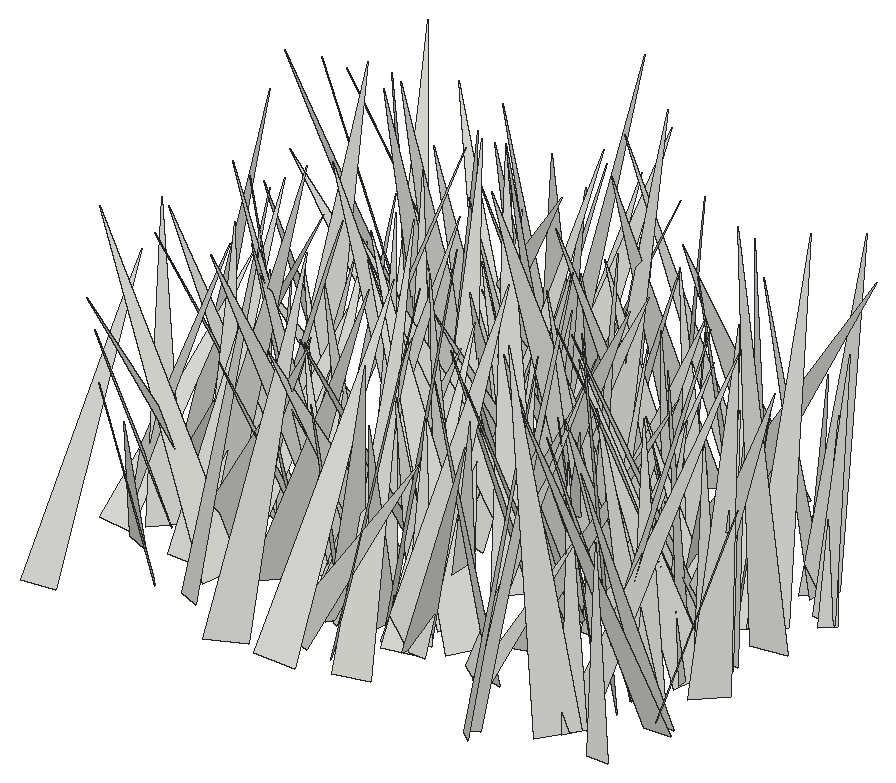
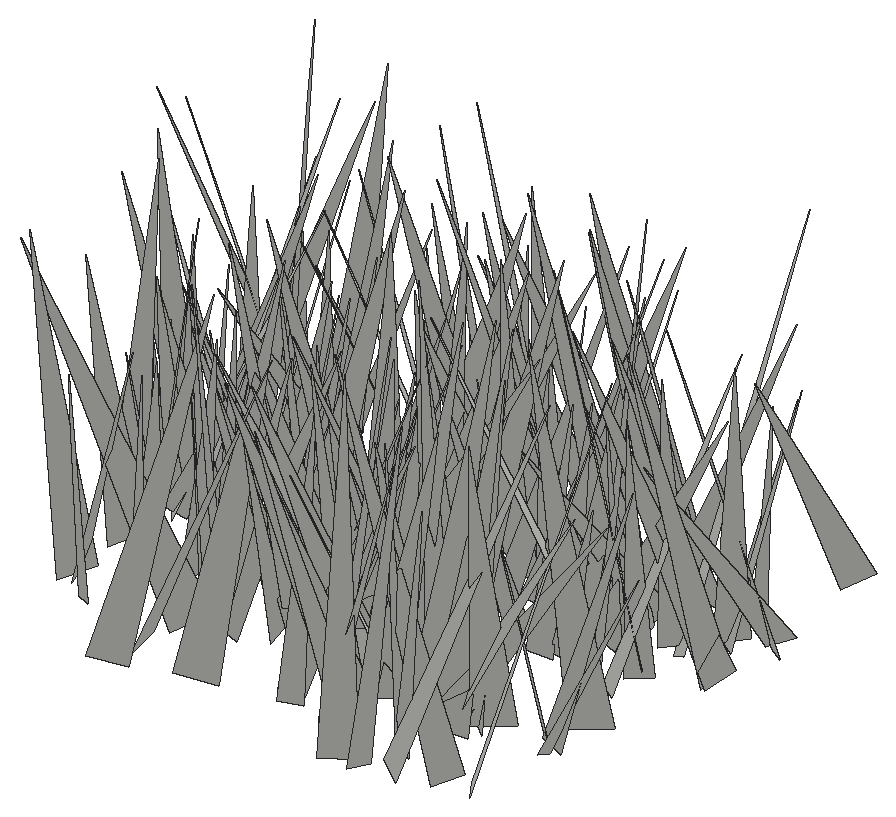
# SketchUp Ruby script. Lengths in inches.
U = 1.inch
M = Sketchup.active_model
def pt(a) = Geom::Point3d.new(a.map { |v| v * U })
def face(e, loops, mat)
  f = e.add_face(loops[0].map { |a| pt(a) })
  loops[1..].each { |l| e.add_face(l.map { |a| pt(a) }).erase! }
  f.material = f.back_material = mat if mat
  f
end
# faces: each face lists its corners as indices into pts; further lists are holes
def faces(e, pts, list, mat = nil) = list.each { |f| face(e, (f[0].is_a?(Array) ? f : [f]).map { |l| l.map { |i| pts[i] } }, mat) }
# xy, xz, yz: faces in a plane at the given z, y or x. An outline is a flat list of corners, or four numbers for a rectangle; further outlines are holes
def ring(l) = l.size == 4 ? [[l[0], l[1]], [l[2], l[1]], [l[2], l[3]], [l[0], l[3]]] : l.each_slice(2).to_a
def flat(e, list, mat, &to3) = list.each { |f| face(e, (f[0].is_a?(Array) ? f : [f]).map { |l| ring(l).map { |u, v| to3.(u, v) } }, mat) }
def xy(e, z, list, mat = nil) = flat(e, list, mat) { |x, y| [x, y, z] }
def xz(e, y, list, mat = nil) = flat(e, list, mat) { |x, z| [x, y, z] }
def yz(e, x, list, mat = nil) = flat(e, list, mat) { |y, z| [x, y, z] }
def lines(e, pts, list) = list.each { |a, b| e.add_line(pt(pts[a]), pt(pts[b])) }
# prism: a flat outline (further loops are holes) pulled along v
def prism(e, loops, v, mat = nil)
  f = face(e, loops, mat); d = Geom::Vector3d.new(v.map { |x| x * U })
  f.pushpull(f.normal.samedirection?(d) ? d.length : -d.length)
end
def box(e, o, s, mat = nil) = prism(e, [[o, [o[0] + s[0], o[1], o[2]], [o[0] + s[0], o[1] + s[1], o[2]], [o[0], o[1] + s[1], o[2]]]], [0, 0, s[2]], mat)
def at(x, y, z, deg = 0) = Geom::Transformation.translation(pt([x, y, z])) * Geom::Transformation.rotation(ORIGIN, Z_AXIS, deg.degrees)
def axes(o, x, y, z) = Geom::Transformation.new([*x, 0, *y, 0, *z, 0, *pt(o).to_a, 1])
def part(name) = M.definitions.add(name)
# library, detail: a bought-in or finely detailed component or shape, given as its bounding box
def library(name, o, s) = part(name).tap { |d| box(d.entities, o, s) }
def detail(e, o, s) = box(e.add_group.entities, o, s)
def put(e, d, t, mat = nil) = e.add_instance(d, t).tap { |i| i.material = mat if mat }
def group(e, t, mat = nil) = e.add_group.tap { |g| g.transformation = t; g.material = mat if mat }.entities
root = M.entities
c1 = part("fur_instance\#9")
p = [[0.8125,0,1.79],[0.67,-0.02,1.48],[0,-0.11,0],[0,0.11,0]]
faces(c1.entities,p,[[0,1,2,3]])
put(root,c1,axes([138.79,360.375,-27.1],[-2.84095,-2.72325,0.75235],[-2.80656,2.8428,-0.30791],[0.32453,0.74533,3.9233]))
put(root,c1,axes([145.17,360.07,-27.1],[2.54302,-4.52945,1.06711],[-4.23804,-1.75205,2.66287],[1.92189,2.12978,4.46004]))
put(root,c1,axes([158.66,360.0625,-27.1],[-0.06677,3.94377,1.582],[4.24655,0.00562,0.16522],[-0.15123,-1.5834,3.94087]))
put(root,c1,axes([143.4,358.59,-27.1],[5.43285,-3.6045,3.64876],[-4.74936,-5.54221,1.59663],[-1.93634,3.48041,6.32132]))
put(root,c1,axes([156.51,360.6,-27.1],[-5.45216,4.70878,2.71596],[5.23215,5.58914,0.81316],[1.47433,-2.42158,7.15803]))
put(root,c1,axes([136.69,362.09,-27.1],[-0.43336,-3.79274,0.22877],[-3.61563,0.48241,1.14868],[1.16807,0.08612,3.64049]))
put(root,c1,axes([135.86,357.625,-27.1],[-4.59878,4.14257,0.47856],[3.69105,4.37512,-2.40275],[1.94062,1.49539,5.70408]))
put(root,c1,axes([146.57,360.7,-27.1],[7.04246,3.4796,1.7186],[3.70112,-7.09298,-0.80545],[-1.16744,-1.49647,7.81378]))
put(root,c1,axes([154.09,358.52,-27.1],[4.5947,4.98178,1.41698],[4.55399,-4.78808,2.06705],[-2.46722,0.43974,6.4542]))
put(root,c1,axes([137.43,365.61,-27.1],[-5.00279,-6.48805,0.18943],[-5.66686,4.48249,3.86684],[3.16501,-2.22958,7.22289]))
put(root,c1,axes([145.65,362.43,-27.1],[5.23742,-3.794,0.7561],[-3.79638,-5.28528,-0.22367],[-0.74406,0.26094,6.46336]))
put(root,c1,axes([145.58,358.55,-27.1],[-1.59566,7.05244,0.57454],[6.94745,1.67322,-1.24356],[1.34162,-0.27674,7.12297]))
put(root,c1,axes([159.07,362.89,-27.1],[-1.75901,-6.72397,0.92553],[-6.70142,1.56883,-1.33876],[-1.07676,1.22044,6.82009]))
put(root,c1,axes([148.83,362.38,-27.1],[5.31861,-1.95589,0.12332],[-1.94358,-5.30997,-0.39374],[-0.25139,-0.32717,5.65315]))
put(root,c1,axes([146.96,362.82,-27.1],[4.83805,-1.95602,0.87332],[-1.75837,-4.85831,-1.14034],[-1.22345,-0.75248,5.09238]))
put(root,c1,axes([152.3,361.39,-27.1],[2.38056,3.51502,0.37387],[3.33138,-2.08023,-1.65431],[1.18197,-1.21634,3.90969]))
put(root,c1,axes([138.8,363.36,-27.1],[2.77166,-6.45652,0.14972],[-5.9267,-2.47813,2.8503],[2.56578,1.25036,6.42219]))
put(root,c1,axes([156.83,361.09,-27.1],[-4.5869,1.43943,1.05541],[1.33614,4.69877,-0.60151],[1.18347,0.27406,4.76967]))
put(root,c1,axes([144.97,363.02,-27.1],[3.60771,1.96245,2.32029],[2.67745,-3.75626,-0.98607],[-1.43745,-2.07119,3.98679]))
put(root,c1,axes([158.9,363.34,-27.1],[-0.82643,-5.48525,0.94931],[-5.54864,0.73423,-0.58792],[-0.44918,1.02229,5.51591]))
put(root,c1,axes([140.375,362.13,-27.1],[-6.66331,2.16551,0.21128],[2.17487,6.60915,0.85019],[-0.06344,-0.87375,6.95459]))
put(root,c1,axes([156.39,363.82,-27.1],[-5.2101,-5.93708,2.74108],[-5.84341,5.80017,1.45611],[2.93548,1.00834,7.76362]))
put(root,c1,axes([136.41,364.17,-27.1],[-3.04266,-3.74721,0.50143],[-3.60797,3.07034,1.05183],[1.12942,-0.28668,4.71094]))
put(root,c1,axes([142.25,365.25,-27.1],[-3.9218,-4.42687,0.35438],[-4.07666,3.77609,2.05553],[1.7617,-1.11678,5.54549]))
put(root,c1,axes([148.41,359.28,-27.1],[0.0768,8.17284,0.16546],[8.06568,-0.10268,1.32775],[-1.3295,-0.15078,8.06464]))
put(root,c1,axes([141.87,362.92,-27.1],[6.48225,-3.39085,0.68777],[-3.4557,-6.41712,0.9323],[-0.17042,1.14593,7.25591]))
put(root,c1,axes([152.53,362.05,-27.1],[-3.42492,-4.02626,1.68032],[-4.34426,2.9504,-1.78518],[-0.40205,2.41841,4.97534]))
put(root,c1,axes([148.8,362.47,-27.1],[-2.37433,3.47563,1.70417],[3.72029,2.6012,-0.12184],[1.06942,-1.33243,4.20745]))
put(root,c1,axes([140.53,360.13,-27.1],[3.83849,6.3713,1.10198],[6.13828,-3.99344,1.70758],[-2.03209,-0.02789,7.23959]))
put(root,c1,axes([144.49,362.77,-27.1],[1.01992,4.1189,1.46608],[4.23417,-0.55549,-1.38501],[1.0893,-1.69737,4.0109]))
put(root,c1,axes([144.74,366.1,-27.1],[-6.04066,-0.63869,2.51357],[0.73038,5.69455,3.20222],[2.48847,-3.22176,5.16172]))
put(root,c1,axes([156.6,364.63,-27.1],[-4.48519,-3.52054,0.94744],[-3.42145,4.58335,0.83384],[1.25916,-0.08621,5.64055]))
put(root,c1,axes([148.57,361.9375,-27.1],[-1.59502,6.99566,2.35908],[7.02793,2.17795,-1.70682],[2.26111,-1.83463,6.96922]))
put(root,c1,axes([146.97,363.15,-27.1],[7.03431,3.48518,2.0857],[3.73576,-7.18871,-0.58711],[-1.59396,-1.46769,7.82836]))
put(root,c1,axes([148.51,365,-27.1],[-2.23247,-5.83337,0.18602],[-5.6892,2.13065,-1.46288],[-1.30221,0.692,6.07224]))
put(root,c1,axes([154.09,358.95,-27.1],[4.35175,7.0169,0.44581],[6.16578,-4.0605,3.72408],[-3.37917,1.6275,7.36925]))
put(root,c1,axes([149.11,364.49,-27.1],[4.27597,-2.96302,0.67606],[-2.94629,-4.32773,-0.33261],[-0.74558,0.10858,5.19161]))
put(root,c1,axes([142.72,363.95,-27.1],[-2.07432,-2.92088,0.84042],[-3.01146,2.11274,-0.09003],[0.41107,0.73854,3.58137]))
put(root,c1,axes([147.82,364.08,-27.1],[-3.6167,2.28369,2.19841],[2.80718,3.85669,0.61192],[1.47241,-1.74341,4.23336]))
put(root,c1,axes([144.92,364.51,-27.1],[1.50784,-3.41822,0.5063],[-3.4457,-1.52893,-0.06057],[-0.26023,0.4385,3.73552]))
put(root,c1,axes([143.4,365.79,-27.1],[1.95168,-6.84621,1.26966],[-6.52036,-2.2596,-2.16121],[-2.44285,0.56154,6.78298]))
put(root,c1,axes([144.15,363.83,-27.1],[4.85202,-3.37562,1.03104],[-3.52041,-4.75453,1.00059],[-0.25408,1.41409,5.82544]))
put(root,c1,axes([156.39,361.89,-27.1],[3.64323,6.95762,0.66244],[6.95502,-3.53547,-1.11744],[0.68929,-1.10109,7.77386]))
put(root,c1,axes([158.26,364.09,-27.1],[4.88732,1.92922,0.49219],[1.99044,-4.76555,-1.08522],[-0.04774,-1.19066,5.14102]))
put(root,c1,axes([134.9,363.39,-27.1],[4.20289,4.66758,0.96744],[4.74909,-3.98911,-1.38552],[0.41036,-1.63927,6.12625]))
put(root,c1,axes([150.39,363.34,-27.1],[-4.97351,5.86998,1.15657],[5.9442,4.67754,1.82131],[-0.6788,-2.04794,7.47498]))
put(root,c1,axes([153.36,365.4,-27.1],[-2.96525,-5.05492,0.58848],[-5.08807,2.93137,-0.45808],[-0.10025,0.73898,5.84252]))
put(root,c1,axes([144.8,362.33,-27.1],[3.51205,7.24819,1.1392],[7.33442,-3.43356,-0.76524],[0.20101,-1.35755,8.01781]))
put(root,c1,axes([156.36,362.51,-27.1],[5.62974,5.25868,1.12192],[5.27805,-5.71471,0.30107],[-1.02693,-0.54292,7.69786]))
put(root,c1,axes([144.77,363.72,-27.1],[-7.94923,-1.56442,0.5472],[-1.62855,7.87073,-1.15603],[0.30767,1.24144,8.0188]))
put(root,c1,axes([157.41,364.3,-27.1],[0.3865,-5.10308,2.42648],[-5.49086,-0.91339,-1.04632],[-1.33405,2.28099,5.00959]))
put(root,c1,axes([151.42,362.09,-27.1],[3.77289,4.9439,0.17652],[4.9129,-3.7705,0.5956],[-0.58026,0.22179,6.19049]))
put(root,c1,axes([139.36,364.74,-27.1],[3.2608,1.42212,0.87051],[1.60342,-3.19897,-0.78016],[-0.45742,-1.07574,3.47082]))
put(root,c1,axes([136.67,363.64,-27.1],[-4.60516,3.74944,1.60687],[3.84875,4.79672,-0.16237],[1.35183,-0.88372,5.93628]))
put(root,c1,axes([140.39,363.18,-27.1],[4.26964,0.47793,1.18834],[0.14194,-4.28676,1.21405],[-1.27296,1.12502,4.1212]))
put(root,c1,axes([138.6,363.51,-27.1],[7.3545,-2.24014,2.18394],[-2.66673,-7.40612,1.38362],[-1.63595,2.00191,7.56257]))
put(root,c1,axes([157.34,364.5,-27.1],[2.70237,-4.42657,2.31196],[-4.83243,-2.98105,-0.05917],[-1.25989,1.93941,5.18593]))
put(root,c1,axes([148.54,361.75,-27.1],[-4.13598,4.27474,0.09369],[4.07434,3.97972,-1.71759],[1.29691,1.13001,5.6947]))
put(root,c1,axes([148.81,364.29,-27.1],[-1.16984,-6.03511,2.92768],[-6.70455,0.96018,-0.69968],[-0.2073,3.00298,6.1075]))
put(root,c1,axes([144.25,364.35,-27.1],[2.31719,-2.3997,1.71249],[-2.74416,-2.55172,0.13746],[-1.07739,1.33819,3.33302]))
put(root,c1,axes([151.54,367.47,-27.1],[6.17469,-3.94346,0.96595],[-3.5616,-6.10514,-2.15707],[-1.94909,-1.33681,7.00177]))
put(root,c1,axes([149.03,364.47,-27.1],[-5.22041,4.31379,0.87725],[4.39805,5.05275,1.32586],[-0.18846,-1.57859,6.64105]))
put(root,c1,axes([143.22,364.55,-27.1],[-3.14224,2.77876,1.0294],[2.91205,3.17344,0.32264],[0.54877,-0.92877,4.18224]))
put(root,c1,axes([138.76,362.15,-27.1],[0.11708,7.08162,0.20269],[7.08451,-0.11681,-0.01106],[0.00771,-0.20285,7.08258]))
put(root,c1,axes([154.96,364.61,-27.1],[-3.71707,-2.68533,1.32909],[-2.9797,3.53518,-1.19076],[0.31439,1.75658,4.42828]))
put(root,c1,axes([146.03,363.85,-27.1],[0.42916,7.00561,1.64499],[7.11073,-0.66598,0.98114],[-1.10544,-1.56418,6.94983]))
put(root,c1,axes([157.76,366.49,-27.1],[-5.95975,2.47486,1.75961],[2.91321,5.75356,1.77469],[0.85695,-2.34763,6.20435]))
put(root,c1,axes([156.88,368.22,-27.1],[-5.73536,-5.62008,0.65862],[-5.46135,5.74328,1.44982],[1.48081,-0.58562,7.89796]))
put(root,c1,axes([135.26,362.63,-27.1],[-2.44099,4.81015,0.04297],[4.37742,2.2412,-2.21652],[1.99437,0.96814,4.91762]))
put(root,c1,axes([151.91,367.38,-27.1],[-0.76321,-4.71965,0.1503],[-4.6984,0.77422,0.45372],[0.47201,0.07524,4.75939]))
put(root,c1,axes([140.65,367.52,-27.1],[-0.18064,-6.52008,0.8881],[-6.57997,0.17015,-0.08916],[-0.06535,0.89016,6.52198]))
put(root,c1,axes([137.96,365.09,-27.1],[3.60386,-3.42869,2.87422],[-4.08632,-4.02533,0.32181],[-1.82182,2.24626,4.96388]))
put(root,c1,axes([151.09,368.03,-27.1],[-0.50575,-5.47671,0.42869],[-5.44927,0.55465,0.65709],[0.69543,0.36321,5.46062]))
put(root,c1,axes([138.57,368.84,-27.1],[-4.91582,-6.36103,2.07601],[-5.8042,5.33544,2.60426],[3.32923,-0.09063,7.60565]))
put(root,c1,axes([137.95,367.01,-27.1],[5.79589,4.16761,1.50359],[4.42839,-5.37215,-2.17978],[0.13803,-2.64446,6.79779]))
put(root,c1,axes([137.8125,369.09,-27.1],[-3.98509,-5.15803,0.00595],[-5.07141,3.91953,1.18509],[0.94137,-0.71992,6.40951]))
put(root,c1,axes([151.54,364.39,-27.1],[5.52796,-0.81869,0.7417],[-1.07099,-4.89962,2.57397],[-0.27083,2.66498,4.96017]))
put(root,c1,axes([140.28,366.42,-27.1],[-1.81659,5.58818,1.87966],[5.39696,0.78429,2.88421],[-2.37355,-2.49359,5.11948]))
put(root,c1,axes([158.39,366.54,-27.1],[-3.98978,2.11987,2.03955],[2.3526,4.36264,0.06771],[1.76604,-1.02247,4.51748]))
put(root,c1,axes([139.4,366.32,-27.1],[1.95895,3.98258,1.69888],[4.26762,-2.09086,-0.01944],[-0.73116,-1.53362,4.43825]))
put(root,c1,axes([135.21,366.08,-27.1],[6.85637,-0.90607,0.05149],[-0.90407,-6.7849,0.99057],[0.07926,0.98874,6.84468]))
put(root,c1,axes([149.9,367.55,-27.1],[-2.91722,-4.26379,0.81225],[-4.33997,2.88016,-0.46811],[0.06569,0.93518,5.14499]))
put(root,c1,axes([158.99,365.89,-27.1],[5.64429,-3.09602,3.33103],[-3.78051,-6.14532,0.69416],[-2.52761,2.27789,6.40012]))
put(root,c1,axes([158.16,367.5625,-27.1],[2.54214,-2.62214,0.84113],[-2.70032,-2.59808,0.06187],[-0.53981,0.64801,3.65161]))
put(root,c1,axes([139.62,363.96,-27.1],[-3.68567,4.23937,0.30212],[3.60627,3.33103,-2.74713],[2.24908,1.60613,4.89997]))
put(root,c1,axes([157.61,368.44,-27.1],[-5.40162,-4.18627,0.13743],[-4.18531,5.38577,-0.4449],[-0.16419,0.43574,6.81941]))
put(root,c1,axes([152.88,368.99,-27.1],[2.25117,-4.50739,0.41367],[-4.42833,-2.28883,-0.84056],[-0.93676,-0.01195,4.96767]))
put(root,c1,axes([137.53,367.66,-27.1],[-2.45808,3.26284,2.53045],[3.74921,2.99751,-0.22312],[1.72995,-1.86016,4.07903]))
put(root,c1,axes([157.625,366.26,-27.1],[-5.30333,-1.20318,1.41609],[-1.56427,5.2022,-1.4382],[1.00301,1.75149,5.24448]))
put(root,c1,axes([141.08,365.625,-27.1],[-2.87102,4.68172,0.40163],[4.57171,2.89185,-1.02921],[1.08596,0.20316,5.39463]))
put(root,c1,axes([142.53,368,-27.1],[1.52627,-4.48364,1.33128],[-4.39877,-0.90019,2.01128],[1.58937,1.81423,4.28804]))
put(root,c1,axes([156.03,368.22,-27.1],[3.29636,-5.4576,1.30622],[-5.51274,-2.86598,1.93739],[1.04942,2.08768,6.07437]))
put(root,c1,axes([141.25,368.57,-27.1],[0.46643,-4.66615,1.44002],[-4.86096,-0.58186,-0.31092],[-0.46655,1.39737,4.67909]))
put(root,c1,axes([135.65,365.86,-27.1],[-6.79191,0.51616,3.38033],[-0.49773,7.28774,-2.11287],[3.3831,2.10844,6.47551]))
put(root,c1,axes([144.375,369.19,-27.1],[4.0303,-5.81988,3.12764],[-5.66664,-4.92868,-1.86917],[-3.39741,1.31665,6.82792]))
put(root,c1,axes([157.97,367.59,-27.1],[-2.87037,3.7349,1.34525],[3.80013,3.06525,-0.40189],[1.14815,-0.80807,4.69329]))
put(root,c1,axes([149.66,369.77,-27.1],[4.03439,-1.67825,0.01541],[-1.64329,-3.95818,-0.85174],[-0.3411,-0.78061,4.28572]))
put(root,c1,axes([154.6,370.03,-27.1],[4.66467,-0.77947,0.02704],[-0.7406,-4.47818,-1.32848],[-0.24456,-1.30606,4.53893]))
put(root,c1,axes([149.18,367.375,-27.1],[-6.71454,4.39928,1.56364],[4.39375,6.8803,-0.4901],[1.57912,-0.43767,8.0124]))
put(root,c1,axes([154.5625,368.39,-27.1],[0.69151,3.97199,1.28395],[4.17346,-0.6309,-0.296],[0.08642,-1.31479,4.02085]))
put(root,c1,axes([157.38,368.57,-27.1],[-1.85647,3.95367,0.8299],[3.82368,1.42492,1.76516],[-1.30372,-1.4508,3.99527]))
put(root,c1,axes([152.96,366.78,-27.1],[2.80201,6.02167,1.40008],[5.6342,-3.12002,2.14317],[-2.54489,-0.27744,6.28638]))
put(root,c1,axes([147.13,370.2,-27.1],[3.33833,-6.51025,0.54896],[-6.14625,-2.92038,2.74304],[2.21549,1.70799,6.78259]))
put(root,c1,axes([152.72,367.97,-27.1],[2.02103,5.13059,0.73898],[5.12624,-1.86067,-1.10143],[0.76856,-1.08099,5.40318]))
put(root,c1,axes([147.71,370.11,-27.1],[-4.43221,4.72995,1.58971],[4.78005,3.41433,3.16821],[-1.43205,-3.24253,5.65503]))
put(root,c1,axes([158.14,368.2,-27.1],[1.43677,3.63281,1.03111],[3.57622,-1.66329,0.8769],[-1.21291,-0.60083,3.80693]))
put(root,c1,axes([151.29,369.41,-27.1],[-5.71627,0.02456,1.51927],[0.09668,5.9079,0.26822],[1.51639,-0.28405,5.71003]))
put(root,c1,axes([140.52,368.21,-27.1],[-1.14245,4.14217,0.46464],[4.01441,0.96381,1.27839],[-1.12161,-0.76952,4.10226]))
put(root,c1,axes([140.23,366.9,-27.1],[5.64336,5.1887,0.30355],[5.15395,-5.64438,0.66329],[-0.67191,0.28398,7.63742]))
put(root,c1,axes([148.5625,370.2,-27.1],[-1.63509,-3.83691,0.93062],[-3.94815,1.58786,-0.39017],[-0.00453,1.00909,4.15248]))
put(root,c1,axes([145.66,371.55,-27.1],[-0.82646,-4.24361,0.01629],[-4.06802,0.79698,1.2278],[1.20816,-0.21938,4.14533]))
put(root,c1,axes([148.79,368.31,-27.1],[-4.40287,4.25609,0.42122],[4.26988,4.40886,0.08361],[0.24458,-0.35298,6.12311]))
put(root,c1,axes([149.28,372.17,-27.1],[5.28612,-6.00356,2.19792],[-5.60526,-5.72373,-2.15328],[-3.07484,0.113,7.70384]))
put(root,c1,axes([146.87,372.67,-27.1],[-4.92711,-3.11526,0.5387],[-2.69685,4.66208,2.29422],[1.64986,-1.68274,5.3589]))
put(root,c1,axes([148.49,368.125,-27.1],[-4.43133,1.84787,0.51045],[1.62369,4.30117,-1.47494],[1.01922,1.18203,4.56901]))
put(root,c1,axes([154.4375,370.26,-27.1],[-2.57629,-2.49445,0.93197],[-2.62206,2.60252,-0.28257],[0.46438,0.85602,3.57488]))
put(root,c1,axes([145.41,368.57,-27.1],[-2.63415,6.93544,1.64719],[7.09873,2.71215,-0.06728],[0.64926,-1.51533,7.41852]))
put(root,c1,axes([154.34,369.67,-27.1],[-5.10853,0.04095,1.59169],[-0.11644,5.32521,-0.51071],[1.58796,0.52222,5.08311]))
put(root,c1,axes([158.49,369.8,-27.1],[-0.94907,-6.99906,3.73248],[-7.88487,0.42284,-1.21201],[-0.8643,3.82797,6.95835]))
put(root,c1,axes([147.15,370.55,-27.1],[-4.76846,2.17787,1.48985],[2.383,4.8757,0.4998],[1.13316,-1.08876,5.21838]))
put(root,c1,axes([149.72,369.47,-27.1],[-6.70794,-1.60484,0.19836],[-1.59675,6.44001,-1.8942],[-0.25542,1.88735,6.63204]))
put(root,c1,axes([137.375,370.49,-27.1],[1.77196,3.84512,1.4323],[4.08534,-1.50774,-1.0065],[0.38272,-1.70823,4.11239]))
put(root,c1,axes([146.46,371.05,-27.1],[0.92533,-3.44435,1.34936],[-3.58141,-1.18238,-0.56215],[-0.92618,1.13092,3.52189]))
put(root,c1,axes([143.45,369.1875,-27.1],[-0.40472,6.25604,0.83945],[6.18781,0.22712,1.29072],[-1.24649,-0.90382,6.13481]))
put(root,c1,axes([145.23,369.95,-27.1],[3.77133,0.16267,0.95437],[-0.10228,-3.74984,1.04331],[-0.96272,1.03561,3.6278]))
put(root,c1,axes([144.08,373.42,-27.1],[4.85347,-3.26157,0.26621],[-3.0891,-4.72355,-1.55255],[-1.07988,-1.1468,5.6377]))
put(root,c1,axes([151.6,369.36,-27.1],[1.45734,4.18221,0.34787],[4.02467,-1.49715,1.13854],[-1.18907,0.05834,4.28]))
put(root,c1,axes([146.98,371,-27.1],[4.06657,-2.17936,1.39694],[-2.40276,-4.14574,0.52683],[-0.9632,1.14071,4.58356]))
put(root,c1,axes([155.69,372.12,-27.1],[-5.52938,-3.456,2.07939],[-3.45701,5.87854,0.57763],[2.07771,0.58365,6.49494]))
put(root,c1,axes([156.48,370.51,-27.1],[3.3556,2.16226,1.21696],[2.08771,-3.56664,0.58052],[-1.34083,-0.14202,3.94948]))
put(root,c1,axes([146.54,371.85,-27.1],[2.73482,-5.11249,1.4467],[-5.08402,-2.04521,2.38319],[1.54377,2.32148,5.28557]))
put(root,c1,axes([156.95,370.53,-27.1],[-1.86757,4.60063,0.33127],[4.58089,1.80817,0.71369],[-0.53944,-0.57279,4.91369]))
put(root,c1,axes([145.72,369.19,-27.1],[2.14003,7.20036,0.0672],[7.19519,-2.14104,0.27303],[-0.28086,0.01341,7.50668]))
put(root,c1,axes([136.58,371.51,-27.1],[-2.68799,6.56885,2.98447],[6.8694,3.30396,-1.08507],[2.20641,-2.2839,7.01411]))
put(root,c1,axes([149.5625,372.04,-27.1],[-0.77235,4.89048,2.70767],[4.92537,1.88806,-2.00519],[2.64368,-2.08884,4.52687]))
put(root,c1,axes([136.89,373.33,-27.1],[-1.73362,-4.79917,0.85478],[-4.86621,1.65027,-0.60395],[-0.28757,1.00633,5.06683]))
put(root,c1,axes([141.82,373.25,-27.1],[7.52805,-0.18805,1.99939],[0.07054,-7.72753,-0.99239],[-2.00698,-0.97696,7.46472]))
put(root,c1,axes([136.75,373.9375,-27.1],[-3.56897,-0.50146,0.42511],[-0.28446,3.29362,1.49696],[0.59267,-1.43888,3.27843]))
put(root,c1,axes([143.22,374.04,-27.1],[-6.0404,2.2493,3.21945],[3.13358,6.3206,1.46334],[2.36747,-2.62704,6.2773]))
put(root,c1,axes([154.05,371.6875,-27.1],[-5.59826,1.4556,0.99849],[1.35798,5.67289,-0.65612],[1.12768,0.39476,5.74707]))
put(root,c1,axes([147.16,373.64,-27.1],[-0.83843,-4.56243,0.7415],[-4.45874,0.59959,-1.35228],[-1.2187,0.94513,4.43735]))
put(root,c1,axes([144.71,371.14,-27.1],[-3.134,4.47853,0.59876],[4.43295,3.18866,-0.64743],[0.8745,-0.1137,5.42771]))
put(root,c1,axes([147.93,372.2,-27.1],[1.92341,3.31368,0.82854],[3.39872,-1.95136,-0.08567],[-0.34002,-0.7604,3.83049]))
put(root,c1,axes([157.47,371.02,-27.1],[-5.92088,3.75972,1.43779],[3.50525,6.07307,-1.44586],[1.97886,0.49178,6.86307]))
put(root,c1,axes([150.875,374.05,-27.1],[-1.01411,-6.0227,1.51425],[-5.97973,0.53295,-1.88497],[-1.67593,1.7428,5.80932]))
put(root,c1,axes([149.61,371.51,-27.1],[1.82525,7.99707,1.79582],[8.16577,-1.93273,0.30716],[-0.70587,-1.67961,8.19697]))
put(root,c1,axes([140.36,374.79,-27.1],[1.08245,-7.41016,1.80762],[-7.58562,-1.23679,-0.52762],[-0.7977,1.70574,7.47019]))
put(root,c1,axes([158.65,372.63,-27.1],[0.70725,4.81258,1.31899],[4.97344,-0.78845,0.21001],[-0.40688,-1.27212,4.85974]))
put(root,c1,axes([159.04,372.35,-27.1],[-3.45785,1.40655,0.59459],[1.25916,3.45892,-0.85969],[0.86397,0.58836,3.63264]))
put(root,c1,axes([141.34,374.77,-27.1],[1.42395,-7.42701,2.10024],[-7.62151,-1.69014,-0.80943],[-1.21824,1.89264,7.51884]))
put(root,c1,axes([150.9375,374.24,-27.1],[4.1746,-2.61988,2.8232],[-2.37692,-5.02847,-1.15163],[-3.03059,0.33503,4.79215]))
put(root,c1,axes([146.28,376,-27.1],[3.38656,-3.48151,1.0277],[-2.77448,-3.38882,-2.33752],[-2.3408,-1.02022,4.25743]))
put(root,c1,axes([148.71,372.5,-27.1],[5.15508,0.33774,1.32609],[0.02228,-5.18864,1.23487],[-1.36825,1.188,5.01637]))
put(root,c1,axes([139.91,373.6875,-27.1],[-4.37552,-5.12362,2.64469],[-5.63456,4.50416,-0.59611],[1.22377,2.41912,6.71129]))
put(root,c1,axes([145.33,374.59,-27.1],[-6.26815,-2.22604,2.13273],[-2.17784,6.6177,0.5065],[2.18193,0.21043,6.63238]))
put(root,c1,axes([140.89,374.47,-27.1],[-3.83855,4.56526,0.77541],[4.17711,2.97899,3.13921],[-1.99865,-2.54191,5.07163]))
put(root,c1,axes([137.43,372.98,-27.1],[2.58432,3.47984,0.90101],[3.42396,-2.72089,0.68775],[-1.09434,-0.29537,4.2796]))
put(root,c1,axes([145.52,372.42,-27.1],[6.4283,2.09347,0.22673],[2.03253,-6.35917,1.08941],[-0.55031,0.96716,6.67224]))
put(root,c1,axes([149,372.08,-27.1],[-5.03448,1.97141,0.87824],[1.57247,4.87743,-1.93439],[1.47821,1.52579,5.04882]))
put(root,c1,axes([150.87,373.99,-27.1],[5.91365,2.78735,2.33328],[2.94924,-6.28377,0.03183],[-2.12497,-0.96423,6.53755]))
put(root,c1,axes([145.21,374.2,-27.1],[5.91491,-0.67607,1.90084],[-0.77835,-6.19702,0.21795],[-1.8613,0.44302,5.94943]))
put(root,c1,axes([152.07,374.27,-27.1],[6.07863,-4.42165,0.21276],[-4.21796,-5.67554,2.55792],[1.3435,2.18706,7.06807]))
put(root,c1,axes([157.35,373.91,-27.1],[-5.62081,-1.07857,0.79033],[-1.22962,5.511,-1.22409],[0.52534,1.35906,5.59093]))
put(root,c1,axes([149.22,372.93,-27.1],[-5.01986,0.40192,1.5189],[-0.17545,4.90978,-1.87904],[1.56135,1.84392,4.67223]))
put(root,c1,axes([157.33,374.03,-27.1],[-5.57842,3.33095,2.99608],[3.28064,6.29556,-0.89096],[3.05108,-0.67911,6.43585]))
put(root,c1,axes([145.85,376.61,-27.1],[0.34868,-5.31048,0.36463],[-5.26358,-0.28954,0.81646],[0.79301,0.41316,5.25892]))
put(root,c1,axes([137.14,377.48,-27.1],[-6.21102,-4.85766,0.88936],[-4.64444,6.23147,1.60082],[1.67841,-0.73247,7.72082]))
put(root,c1,axes([149.47,377.3,-27.1],[2.6009,-7.25193,0.96085],[-7.2129,-2.71231,-0.94648],[-1.21974,0.57558,7.64587]))
put(root,c1,axes([149.94,376.2,-27.1],[4.17117,1.8451,1.43695],[2.27213,-3.89306,-1.59669],[-0.55375,-2.07548,4.27243]))
put(root,c1,axes([156,375.38,-27.1],[-1.72893,-3.46771,1.76985],[-3.62718,2.13831,0.64633],[1.41454,1.24466,3.82053]))
put(root,c1,axes([141.12,373.74,-27.1],[-6.11447,-3.98639,0.59028],[-3.68819,5.10346,-3.73879],[-1.62389,3.41906,6.26894]))
put(root,c1,axes([143.76,373.97,-27.1],[-4.22823,5.63878,0.60494],[5.64653,4.11564,1.10357],[-0.52773,-1.14251,6.96102]))
put(root,c1,axes([144.16,377.13,-27.1],[-4.57132,-4.01454,0.83204],[-3.89365,4.6413,1.00178],[1.28384,-0.21818,6.00082]))
put(root,c1,axes([138.18,377.46,-27.1],[1.13503,-7.67663,0.6742],[-6.50823,-0.58999,4.2389],[4.12651,1.18099,6.50005]))
put(root,c1,axes([152.65,378.23,-27.1],[3.73251,-5.71066,0.85994],[-5.41751,-3.81707,-1.83396],[-2.00044,-0.31799,6.57114]))
put(root,c1,axes([139.35,373.45,-27.1],[-4.20767,6.2047,0.57896],[6.20765,4.23458,-0.26697],[0.54635,-0.32858,7.49209]))
put(root,c1,axes([144.33,372.9375,-27.1],[3.4696,4.95294,0.18512],[4.68916,-3.35343,1.83583],[-1.60551,0.90933,5.7619]))
put(root,c1,axes([141.11,376.27,-27.1],[5.21956,1.10973,1.69595],[1.36173,-5.39042,-0.66376],[-1.50115,-1.03121,5.29478]))
put(root,c1,axes([154.13,374.8,-27.1],[-5.50715,-0.70612,1.61288],[-1.08889,5.52799,-1.29784],[1.38358,1.53996,5.39842]))
put(root,c1,axes([140.17,378.2,-27.1],[-4.57477,-6.03245,0.25242],[-6.03633,4.57654,-0.02819],[0.13005,0.21817,7.57088]))
put(root,c1,axes([146.06,372.3,-27.1],[7.29611,1.84526,3.54482],[-0.04664,-7.33917,3.91643],[-3.99607,3.45479,6.4265]))
put(root,c1,axes([152.49,376.5,-27.1],[-7.29173,-1.24054,0.1592],[-1.24954,7.26646,-0.60898],[0.05425,0.6271,7.37139]))
put(root,c1,axes([144.55,374.81,-27.1],[-2.83058,6.09964,1.95872],[5.76034,3.3604,-2.14023],[2.80369,-0.74599,6.37473]))
put(root,c1,axes([142.11,378.64,-27.1],[2.97455,-6.14482,0.55918],[-6.16848,-2.94679,0.43089],[0.14598,0.69067,6.8133]))
put(root,c1,axes([140.75,376.83,-27.1],[1.70203,4.17643,2.24286],[4.55719,-2.09788,0.44817],[-1.30578,-1.87783,4.48761]))
put(root,c1,axes([143.98,375.91,-27.1],[0.03547,5.69131,1.501],[5.73382,0.30561,-1.29426],[1.32938,-1.46999,5.5423]))
put(root,c1,axes([144.48,376.14,-27.1],[-6.24639,-1.28271,0.8155],[-1.43317,6.11916,-1.35263],[0.50635,1.49608,6.23162]))
put(root,c1,axes([141.22,378.61,-27.1],[5.81845,-0.62274,2.18855],[-0.03101,-6.03017,-1.6334],[-2.27522,-1.51035,5.61909]))
